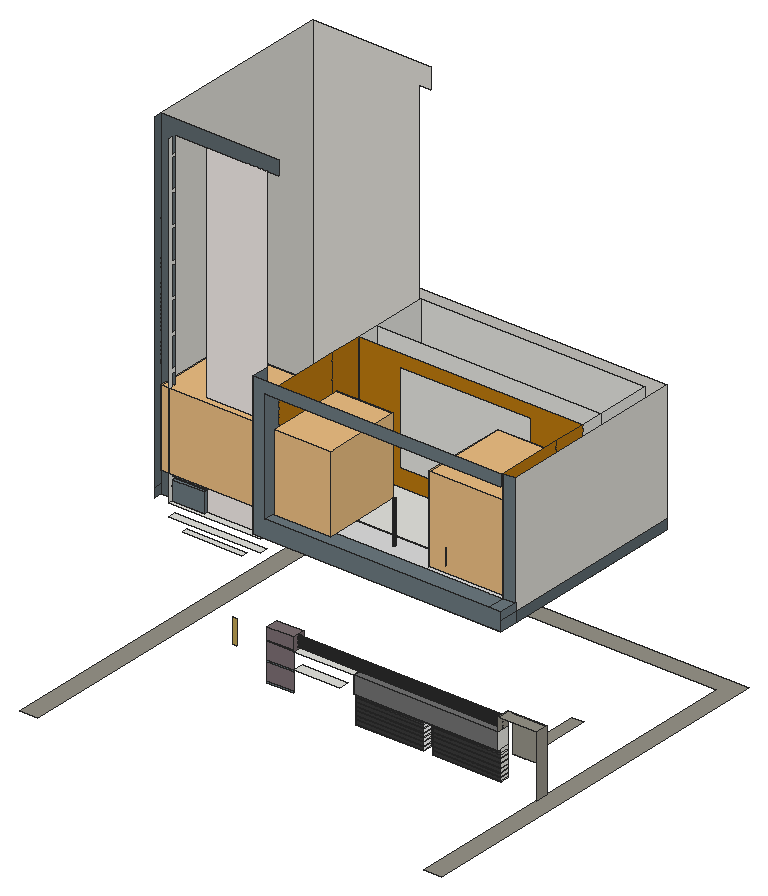
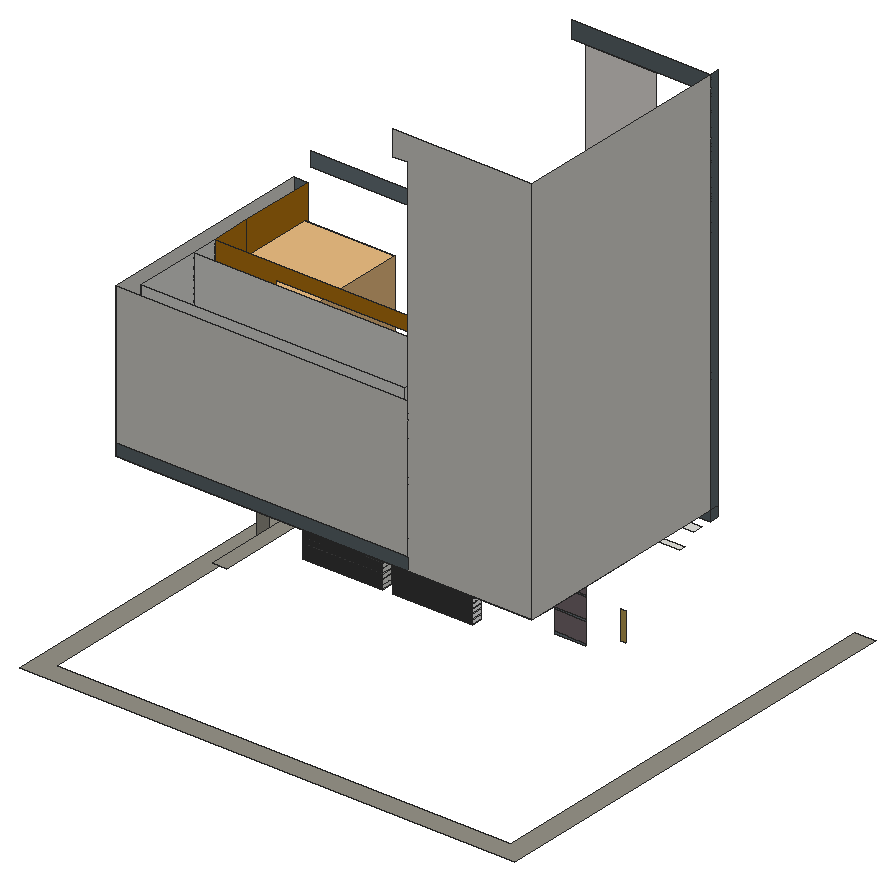
# SketchUp Ruby script. Lengths in inches.
U = 1.inch
M = Sketchup.active_model
def pt(a) = Geom::Point3d.new(a.map { |v| v * U })
def face(e, loops, mat)
  f = e.add_face(loops[0].map { |a| pt(a) })
  loops[1..].each { |l| e.add_face(l.map { |a| pt(a) }).erase! }
  f.material = f.back_material = mat if mat
  f
end
# faces: each face lists its corners as indices into pts; further lists are holes
def faces(e, pts, list, mat = nil) = list.each { |f| face(e, (f[0].is_a?(Array) ? f : [f]).map { |l| l.map { |i| pts[i] } }, mat) }
# xy, xz, yz: faces in a plane at the given z, y or x. An outline is a flat list of corners, or four numbers for a rectangle; further outlines are holes
def ring(l) = l.size == 4 ? [[l[0], l[1]], [l[2], l[1]], [l[2], l[3]], [l[0], l[3]]] : l.each_slice(2).to_a
def flat(e, list, mat, &to3) = list.each { |f| face(e, (f[0].is_a?(Array) ? f : [f]).map { |l| ring(l).map { |u, v| to3.(u, v) } }, mat) }
def xy(e, z, list, mat = nil) = flat(e, list, mat) { |x, y| [x, y, z] }
def xz(e, y, list, mat = nil) = flat(e, list, mat) { |x, z| [x, y, z] }
def yz(e, x, list, mat = nil) = flat(e, list, mat) { |y, z| [x, y, z] }
def lines(e, pts, list) = list.each { |a, b| e.add_line(pt(pts[a]), pt(pts[b])) }
# prism: a flat outline (further loops are holes) pulled along v
def prism(e, loops, v, mat = nil)
  f = face(e, loops, mat); d = Geom::Vector3d.new(v.map { |x| x * U })
  f.pushpull(f.normal.samedirection?(d) ? d.length : -d.length)
end
def box(e, o, s, mat = nil) = prism(e, [[o, [o[0] + s[0], o[1], o[2]], [o[0] + s[0], o[1] + s[1], o[2]], [o[0], o[1] + s[1], o[2]]]], [0, 0, s[2]], mat)
def at(x, y, z, deg = 0) = Geom::Transformation.translation(pt([x, y, z])) * Geom::Transformation.rotation(ORIGIN, Z_AXIS, deg.degrees)
def axes(o, x, y, z) = Geom::Transformation.new([*x, 0, *y, 0, *z, 0, *pt(o).to_a, 1])
def part(name) = M.definitions.add(name)
# library, detail: a bought-in or finely detailed component or shape, given as its bounding box
def library(name, o, s) = part(name).tap { |d| box(d.entities, o, s) }
def detail(e, o, s) = box(e.add_group.entities, o, s)
def put(e, d, t, mat = nil) = e.add_instance(d, t).tap { |i| i.material = mat if mat }
def group(e, t, mat = nil) = e.add_group.tap { |g| g.transformation = t; g.material = mat if mat }.entities
root = M.entities
M.materials.add("[0130_Gainsboro]").color = [220, 220, 220]
M.materials.add("[Asphalt New]").color = [124, 111, 115]
M.materials.add("[Blinds Cloth Horizontal]").color = [192, 163, 85]
M.materials.add("[Blinds Wood Light]").color = [186, 120, 16]
M.materials.add("[Color M00]").color = [255, 255, 255]
M.materials.add("[Color M05]").color = [114, 114, 114]
M.materials.add("[Color M06]").color = [86, 86, 86]
M.materials.add("[Color M07]").color = [58, 58, 58]
M.materials.add("[Formica Graystone]").color = [149, 146, 135]
M.materials.add("[Formica Laminate Dark]").color = [50, 53, 60]
M.materials.add("[Formica Speckled Grey]").color = [107, 120, 127]
M.materials.add("[Formica Speckled Grey]1").color = [94, 105, 111]
M.materials.add("[Terrazzo Tile Light]").color = [219, 217, 210]
M.materials.add("[White Square Tile]").color = [240, 234, 230]
c1 = library("chau cay",[-24.34,-109.24,0],[56.46,62.58,79.69])
c2 = library("Sem+nome",[-20.92,-6.25,0],[92.79,42.83,52.11])
xy(root,41.8125,[[0,0,9.63,0,9.63,200.71,221.32,200.71,221.32,0,230.95,0,230.95,210.34,0,210.34]],"[Formica Graystone]")
xy(root,42.59,[[200.125,79.26,200.1875,83.94]])
xy(root,42.59,[[162.78,79.26,200.125,83.94]],"[Color M07]")
xy(root,42.84,[[120.8,79.26,158.09,83.94]],"[Color M07]")
xy(root,42.9,[[162.78,79.26,200.125,83.94]],"[Color M07]")
xy(root,43.27,[[120.8,79.26,158.09,83.94]],"[Color M07]")
xy(root,44.66,[[162.78,79.26,200.125,83.94]],"[Color M07]")
xy(root,44.96,[[162.78,79.26,200.125,83.94]],"[Color M07]")
xy(root,45.03,[[120.8,79.26,158.09,83.94]],"[Color M07]")
xy(root,45.46,[[120.8,79.26,158.09,83.94]],"[Color M07]")
xy(root,46.72,[[162.78,79.26,200.125,83.94]],"[Color M07]")
xy(root,47.21,[[162.78,79.26,200.125,83.94]],"[Color M07]")
xy(root,47.22,[[120.8,79.26,158.09,83.94]],"[Color M07]")
xy(root,47.65,[[120.8,79.26,158.09,83.94]],"[Color M07]")
xy(root,48.97,[[162.78,79.26,200.125,83.94]],"[Color M07]")
xy(root,49.41,[[120.8,79.26,158.09,83.94]],"[Color M07]")
xy(root,49.59,[[162.78,79.26,200.125,83.94]],"[Color M07]")
xy(root,49.84,[[120.8,79.26,158.09,83.94]],"[Color M07]")
xy(root,51.34,[[162.78,79.26,200.125,83.94]],"[Color M07]")
xy(root,51.59,[[120.8,79.26,158.09,83.94]],"[Color M07]")
xy(root,51.96,[[162.78,79.26,200.125,83.94]],"[Color M07]")
xy(root,52.02,[[120.8,79.26,158.09,83.94]],"[Color M07]")
xy(root,53.72,[[162.78,79.26,200.125,83.94]],"[Color M07]")
xy(root,53.78,[[120.8,79.26,158.09,83.94]],"[Color M07]")
xy(root,54.21,[[120.8,79.26,158.09,83.94],[162.78,79.26,200.125,83.94]],"[Color M07]")
xy(root,55.3125,[[202.93,83.94,209.59,124.55]],"[Formica Graystone]")
xy(root,55.97,[[120.8,79.26,158.09,83.94],[162.78,79.26,200.125,83.94]],"[Color M07]")
xy(root,56.67,[[120.8,79.26,158.09,83.94],[162.78,79.26,200.125,83.94]],"[Color M07]")
xy(root,58.88,[[88.1,77.29,113.16,83.29],[120.8,79.26,158.09,83.94],[162.78,79.26,200.125,83.94]])
xy(root,58.88,[[120.8,77.29,200.125,79.26]],"[Color M05]")
xy(root,68,[[88.1,77.29,120.8,83.94]])
xy(root,68,[[120.8,77.29,200.125,83.94]],"[Color M05]")
xy(root,75.3125,[[73.48,77.29,88.1,83.94]],"[Asphalt New]")
xy(root,75.3125,[[200.125,77.29,221.32,83.94]],"[Formica Graystone]")
xy(root,105.34,[[27.2,77.29,59.83,80.42]])
xy(root,112.0625,[[97.58,124.55,186.72,127.86]])
xy(root,113.3,[[22.92,72.92,73.48,77.29]])
xy(root,120,[[22.92,72.92,73.48,72.92,73.48,77.29,40.57,77.29,40.57,75.48,22.92,75.48],[22.92,75.48,40.57,77.29]])
xy(root,124.8125,[[90.48,86.18,89.1875,86.35,87.98,86.85,86.95,87.65,86.15,88.68,85.65,89.89,85.48,91.18,85.65,92.48,86.15,93.68,86.95,94.72,87.98,95.51,89.1875,96.01,90.48,96.18,91.78,96.01,92.98,95.51,94.02,94.72,94.8125,93.68,95.3125,92.48,95.48,91.18,95.3125,89.89,94.8125,88.68,94.02,87.65,92.98,86.85,91.78,86.35],[138.67,86.18,137.375,86.35,136.17,86.85,135.13,87.65,134.34,88.68,133.84,89.89,133.67,91.18,133.84,92.48,134.34,93.68,135.13,94.72,136.17,95.51,137.375,96.01,138.67,96.18,139.96,96.01,141.17,95.51,142.21,94.72,143,93.68,143.5,92.48,143.67,91.18,143.5,89.89,143,88.68,142.21,87.65,141.17,86.85,139.96,86.35],[185.98,86.18,184.6875,86.35,183.48,86.85,182.45,87.65,181.65,88.68,181.15,89.89,180.98,91.18,181.15,92.48,181.65,93.68,182.45,94.72,183.48,95.51,184.6875,96.01,185.98,96.18,187.28,96.01,188.48,95.51,189.52,94.72,190.3125,93.68,190.8125,92.48,190.98,91.18,190.8125,89.89,190.3125,88.68,189.52,87.65,188.48,86.85,187.28,86.35],[15.28,124.55,21.94,129.24],[21.94,124.55,202.93,129.24],
  [202.93,124.55,209.59,129.24],[15.28,129.24,21.94,174.54],[21.94,129.24,202.93,174.54],[202.93,129.24,209.59,181.19],[15.28,174.54,202.93,181.19]])
xy(root,124.8125,[[73.48,67.6,209.59,77.29]],"[Formica Speckled Grey]")
xy(root,124.8125,[[[73.48,77.29,209.59,124.55],[90.48,86.18,91.78,86.35,92.98,86.85,94.02,87.65,94.8125,88.68,95.3125,89.89,95.48,91.18,95.3125,92.48,94.8125,93.68,94.02,94.72,92.98,95.51,91.78,96.01,90.48,96.18,89.1875,96.01,87.98,95.51,86.95,94.72,86.15,93.68,85.65,92.48,85.48,91.18,85.65,89.89,86.15,88.68,86.95,87.65,87.98,86.85,89.1875,86.35],[185.98,86.18,187.28,86.35,188.48,86.85,189.52,87.65,190.3125,88.68,190.8125,89.89,190.98,91.18,190.8125,92.48,190.3125,93.68,189.52,94.72,188.48,95.51,187.28,96.01,185.98,96.18,184.6875,96.01,183.48,95.51,182.45,94.72,181.65,93.68,181.15,92.48,180.98,91.18,181.15,89.89,181.65,88.68,182.45,87.65,183.48,86.85,184.6875,86.35],[138.67,86.18,139.96,86.35,141.17,86.85,142.21,87.65,143,88.68,143.5,89.89,143.67,91.18,143.5,92.48,143,93.68,142.21,94.72,141.17,95.51,139.96,96.01,138.67,96.18,137.375,96.01,136.17,95.51,135.13,94.72,134.34,93.68,133.84,92.48,133.67,91.18,133.84,89.89,134.34,88.68,135.13,87.65,136.17,86.85,137.375,86.35]]],"[Formica Speckled Grey]1")
xy(root,130.3125,[[80.125,91.25,202.95,131.65],[80.125,131.65,202.95,143.96],[80.125,143.96,202.95,174.55]])
xy(root,130.5,[[22.92,75.48,40.57,77.29]],"[Formica Speckled Grey]")
xy(root,132.27,[[22.92,75.48,40.57,77.29]],"[Formica Speckled Grey]")
xy(root,134.5,[[104.45,84,104.25,84.02,104.07,84.1,103.92,84.22,103.8,84.375,103.72,84.55,103.7,84.75,103.72,84.94,103.8,85.125,103.92,85.28,104.07,85.4,104.25,85.47,104.45,85.5,104.64,85.47,104.82,85.4,104.98,85.28,105.1,85.125,105.17,84.94,105.2,84.75,105.17,84.55,105.1,84.375,104.98,84.22,104.82,84.1,104.64,84.02],[137.32,84,137.13,84.02,136.95,84.1,136.79,84.22,136.67,84.375,136.6,84.55,136.57,84.75,136.6,84.94,136.67,85.125,136.79,85.28,136.95,85.4,137.13,85.47,137.32,85.5,137.52,85.47,137.7,85.4,137.85,85.28,137.97,85.125,138.05,84.94,138.07,84.75,138.05,84.55,137.97,84.375,137.85,84.22,137.7,84.1,137.52,84.02],[166.51,84,166.32,84.02,166.13,84.1,165.98,84.22,165.86,84.375,165.79,84.55,165.76,84.75,165.79,84.94,165.86,85.125,165.98,85.28,166.13,85.4,166.32,85.47,166.51,85.5,166.7,85.47,166.88,85.4,167.04,85.28,167.16,85.125,167.23,84.94,167.26,84.75,167.23,84.55,167.16,84.375,167.04,84.22,166.88,84.1,166.7,84.02]])
xy(root,134.5,[[[80.125,77.29,202.95,91.25],[166.51,84,166.32,84.02,166.13,84.1,165.98,84.22,165.86,84.375,165.79,84.55,165.76,84.75,165.79,84.94,165.86,85.125,165.98,85.28,166.13,85.4,166.32,85.47,166.51,85.5,166.7,85.47,166.88,85.4,167.04,85.28,167.16,85.125,167.23,84.94,167.26,84.75,167.23,84.55,167.16,84.375,167.04,84.22,166.88,84.1,166.7,84.02],[137.32,84,137.13,84.02,136.95,84.1,136.79,84.22,136.67,84.375,136.6,84.55,136.57,84.75,136.6,84.94,136.67,85.125,136.79,85.28,136.95,85.4,137.13,85.47,137.32,85.5,137.52,85.47,137.7,85.4,137.85,85.28,137.97,85.125,138.05,84.94,138.07,84.75,138.05,84.55,137.97,84.375,137.85,84.22,137.7,84.1,137.52,84.02],[104.45,84,104.25,84.02,104.07,84.1,103.92,84.22,103.8,84.375,103.72,84.55,103.7,84.75,103.72,84.94,103.8,85.125,103.92,85.28,104.07,85.4,104.25,85.47,104.45,85.5,104.64,85.47,104.82,85.4,104.98,85.28,105.1,85.125,105.17,84.94,105.2,84.75,105.17,84.55,105.1,84.375,104.98,84.22,104.82,84.1,104.64,84.02]]],"[0130_Gainsboro]")
xy(root,134.5,[[80.125,67.6,202.95,77.29],[202.95,67.6,209.59,77.29]],"[Formica Speckled Grey]")
xz(root,67.6,[[73.48,124.8125,209.59,124.8125,209.59,134.5,80.125,134.5,80.125,195.875,209.59,195.875,209.59,202.375,73.48,202.375]],"[Formica Speckled Grey]")
xz(root,75.48,[[22.92,120,40.57,130.5],[22.92,132.27,40.57,146.25]],"[Formica Speckled Grey]")
xz(root,77.29,[[22.92,120,40.57,130.5],[22.92,132.27,40.57,146.25]])
xz(root,77.29,[[73.48,48.75,88.1,57.875],[73.48,58.88,88.1,68],[73.48,68.86,88.1,75.3125]],"[Asphalt New]")
xz(root,77.29,[[120.8,58.88,200.125,68]],"[Color M05]")
xz(root,77.29,[[22.92,130.5,40.57,132.27]],"[Formica Laminate Dark]")
xz(root,77.29,[[73.48,47.5625,88.1,48.75],[73.48,57.875,88.1,58.88],[73.48,68,88.1,68.86],[202.95,134.5,209.59,195.875]],"[Formica Speckled Grey]")
xz(root,77.29,[[15.28,120,15.28,306.8125,80.125,306.8125,80.125,298.85,22.92,298.85,22.92,120]],"[Formica Speckled Grey]1")
xz(root,77.29,[[40.57,120,73.48,298.85]],"[White Square Tile]")
xz(root,79.26,[[162.78,42.9,200.125,44.66],[120.8,43.27,158.09,45.03],[162.78,44.96,200.125,46.72],[120.8,45.46,158.09,47.22],[162.78,47.21,200.125,48.97],
  [120.8,47.65,158.09,49.41],[162.78,49.59,200.125,51.34],[120.8,49.84,158.09,51.59],[162.78,51.96,200.125,53.72],[120.8,52.02,158.09,53.78],
  [120.8,54.21,158.09,55.97],[162.78,54.21,200.125,55.97],[120.8,56.67,158.09,58.88],[162.78,56.67,200.125,58.88]],"[Color M07]")
xz(root,80.42,[[52.45,57.88,54.7,71.19]],"[Blinds Cloth Horizontal]")
xz(root,83.94,[[120.8,58.88,200.125,68]],"[Color M05]")
xz(root,83.94,[[162.78,42.9,200.125,44.66],[120.8,43.27,158.09,45.03],[162.78,44.96,200.125,46.72],[120.8,45.46,158.09,47.22],[162.78,47.21,200.125,48.97],
  [120.8,47.65,158.09,49.41],[162.78,49.59,200.125,51.34],[120.8,49.84,158.09,51.59],[162.78,51.96,200.125,53.72],[120.8,52.02,158.09,53.78],
  [120.8,54.21,158.09,55.97],[162.78,54.21,200.125,55.97],[120.8,56.67,158.09,58.88],[162.78,56.67,200.125,58.88]],"[Color M07]")
xz(root,83.94,[[202.93,55.3125,221.32,75.3125]],"[Formica Graystone]")
xz(root,91.25,[[80.125,130.3125,202.95,134.5]])
xz(root,131.65,[[[80.125,130.3125,202.95,195.875],[102.7,139.62,174.38,189.18]]],"[Blinds Wood Light]")
xz(root,143.96,[[80.125,130.3125,202.95,195.875]])
xz(root,174.55,[[80.125,130.3125,202.95,195.875]])
xz(root,181.19,[[73.48,124.8125,209.59,130.3125]],"[Formica Speckled Grey]1")
xz(root,181.19,[[15.28,124.8125,15.28,306.8125,80.125,306.8125,80.125,295.4375,73.48,295.4375,73.48,124.8125],[73.48,130.3125,209.59,195.875]],"[Terrazzo Tile Light]")
yz(root,15.28,[[72.92,120,77.29,124.8125],[72.92,124.8125,77.29,306.8125]],"[Formica Speckled Grey]1")
yz(root,15.28,[[77.29,124.8125,181.19,306.8125]],"[Terrazzo Tile Light]")
yz(root,22.92,[[72.92,120,75.48,120,75.48,130.5,77.29,130.5,77.29,132.27,75.48,132.27,75.48,146.25,77.29,146.25,77.29,148.25,75.48,148.25,75.48,164,77.29,164,77.29,166.81,75.48,166.81,75.48,182.5625,77.29,182.5625,77.29,184.81,75.48,184.81,75.48,200.5625,77.29,200.5625,77.29,202.43,75.48,202.43,75.48,218.1875,77.29,218.1875,77.29,220,75.48,220,75.48,235.75,77.29,235.75,77.29,237.75,75.48,237.75,75.48,253.5,77.29,253.5,77.29,255.31,75.48,255.31,75.48,271.0625,77.29,271.0625,77.29,272.68,75.48,272.68,75.48,288.4375,77.29,288.4375,77.29,290.11,75.48,290.11,75.48,298.85,72.92,298.85],[75.48,132.27,77.29,146.25]])
yz(root,22.92,[[75.48,120,77.29,130.5]],"[Formica Speckled Grey]1")
yz(root,40.57,[[75.48,120,77.29,130.5],[75.48,132.27,77.29,146.25]],"[Formica Speckled Grey]")
yz(root,73.48,[[67.6,124.8125,77.29,202.375]],"[Formica Speckled Grey]")
yz(root,80.125,[[131.65,130.3125,143.96,195.875],[143.96,130.3125,174.55,195.875]])
yz(root,80.125,[[91.25,130.3125,131.65,130.3125,131.65,195.875,113.38,195.875,113.38,134.5,91.25,134.5],[[77.29,134.5,113.38,195.875],[84.34,157.04,84.16,157.06,83.99,157.13,83.85,157.24,83.74,157.38,83.67,157.54,83.65,157.72,83.67,157.9,83.74,158.07,83.85,158.21,83.99,158.32,84.16,158.39,84.34,158.41,84.51,158.39,84.68,158.32,84.82,158.21,84.93,158.07,85,157.9,85.02,157.72,85,157.54,84.93,157.38,84.82,157.24,84.68,157.13,84.51,157.06],[84.34,151.97,84.16,152,83.99,152.06,83.85,152.17,83.74,152.32,83.67,152.48,83.65,152.66,83.67,152.84,83.74,153,83.85,153.15,83.99,153.26,84.16,153.32,84.34,153.35,84.51,153.32,84.68,153.26,84.82,153.15,84.93,153,85,152.84,85.02,152.66,85,152.48,84.93,152.32,84.82,152.17,84.68,152.06,84.51,152],[84.34,154.47,84.16,154.5,83.99,154.56,83.85,154.67,83.74,154.82,83.67,154.98,83.65,155.16,83.67,155.34,83.74,155.5,83.85,155.65,83.99,155.76,84.16,155.82,84.34,155.85,84.51,155.82,84.68,155.76,84.82,155.65,84.93,155.5,85,155.34,85.02,155.16,85,154.98,84.93,154.82,84.82,154.67,84.68,154.56,84.51,154.5],[84.14,139.71,83.98,139.73,83.83,139.79,83.7,139.89,83.6,140.02,83.54,140.17,83.52,140.33,83.54,140.49,83.6,140.64,83.7,140.77,83.83,140.87,83.98,140.93,84.14,140.96,84.3,140.93,84.45,140.87,84.58,140.77,84.68,140.64,84.74,140.49,84.77,140.33,84.74,140.17,84.68,140.02,84.58,139.89,84.45,139.79,84.3,139.73],[84.14,142.77,83.98,142.79,83.83,142.85,83.7,142.95,83.6,143.08,83.54,143.23,83.52,143.39,83.54,143.56,83.6,143.71,83.7,143.84,83.83,143.93,83.98,144,84.14,144.02,84.3,144,84.45,143.93,84.58,143.84,84.68,143.71,84.74,143.56,84.77,143.39,84.74,143.23,84.68,143.08,84.58,142.95,84.45,142.85,84.3,142.79],[84.31,136.76,84.15,136.78,84,136.84,83.87,136.94,83.77,137.07,83.7,137.22,83.68,137.39,83.7,137.55,83.77,137.7,83.87,137.83,84,137.93,84.15,137.99,84.31,138.01,84.47,137.99,84.62,137.93,84.75,137.83,84.85,137.7,84.91,137.55,84.93,137.39,84.91,137.22,84.85,137.07,84.75,136.94,84.62,136.84,84.47,136.78],[84.31,145.95,84.15,145.97,84,146.03,83.87,146.13,83.77,146.26,83.7,146.41,83.68,146.57,83.7,146.74,83.77,146.89,83.87,147.02,84,147.11,84.15,147.18,84.31,147.2,84.47,147.18,84.62,147.11,84.75,147.02,84.85,146.89,84.91,146.74,84.93,146.57,84.91,146.41,84.85,146.26,84.75,146.13,84.62,146.03,84.47,145.97],[84.31,149.39,84.15,149.41,84,149.47,83.87,149.57,83.77,149.7,83.7,149.85,83.68,150.01,83.7,150.17,83.77,150.32,83.87,150.45,84,150.55,84.15,150.61,84.31,150.64,84.47,150.61,84.62,150.55,84.75,150.45,84.85,150.32,84.91,150.17,84.93,150.01,84.91,149.85,84.85,149.7,84.75,149.57,84.62,149.47,84.47,149.41]]],"[Blinds Wood Light]")
yz(root,80.125,[[67.6,134.5,77.29,195.875]],"[Formica Speckled Grey]")
yz(root,88.1,[[80.61,68.75,80.4375,68.78,80.27,68.84,80.13,68.95,80.02,69.1,79.95,69.26,79.93,69.4375,79.95,69.62,80.02,69.78,80.13,69.93,80.27,70.03,80.4375,70.1,80.61,70.125,80.79,70.1,80.96,70.03,81.1,69.93,81.21,69.78,81.28,69.62,81.3,69.4375,81.28,69.26,81.21,69.1,81.1,68.95,80.96,68.84,80.79,68.78],[80.51,70.85,80.33,70.875,80.17,70.94,80.02,71.05,79.91,71.19,79.85,71.36,79.82,71.54,79.85,71.72,79.91,71.88,80.02,72.02,80.17,72.13,80.33,72.2,80.51,72.23,80.6875,72.2,80.85,72.13,81,72.02,81.1,71.88,81.17,71.72,81.2,71.54,81.17,71.36,81.1,71.19,81,71.05,80.85,70.94,80.6875,70.875],[80.48,72.98,80.25,73.01,80.04,73.1,79.86,73.24,79.72,73.42,79.64,73.63,79.61,73.86,79.64,74.08,79.72,74.3,79.86,74.48,80.04,74.62,80.25,74.7,80.48,74.73,80.71,74.7,80.92,74.62,81.1,74.48,81.24,74.3,81.33,74.08,81.36,73.86,81.33,73.63,81.24,73.42,81.1,73.24,80.92,73.1,80.71,73.01]])
yz(root,88.1,[[[77.29,68,83.94,75.3125],[80.48,72.98,80.25,73.01,80.04,73.1,79.86,73.24,79.72,73.42,79.64,73.63,79.61,73.86,79.64,74.08,79.72,74.3,79.86,74.48,80.04,74.62,80.25,74.7,80.48,74.73,80.71,74.7,80.92,74.62,81.1,74.48,81.24,74.3,81.33,74.08,81.36,73.86,81.33,73.63,81.24,73.42,81.1,73.24,80.92,73.1,80.71,73.01],[80.61,68.75,80.4375,68.78,80.27,68.84,80.13,68.95,80.02,69.1,79.95,69.26,79.93,69.4375,79.95,69.62,80.02,69.78,80.13,69.93,80.27,70.03,80.4375,70.1,80.61,70.125,80.79,70.1,80.96,70.03,81.1,69.93,81.21,69.78,81.28,69.62,81.3,69.4375,81.28,69.26,81.21,69.1,81.1,68.95,80.96,68.84,80.79,68.78],[80.51,70.85,80.33,70.875,80.17,70.94,80.02,71.05,79.91,71.19,79.85,71.36,79.82,71.54,79.85,71.72,79.91,71.88,80.02,72.02,80.17,72.13,80.33,72.2,80.51,72.23,80.6875,72.2,80.85,72.13,81,72.02,81.1,71.88,81.17,71.72,81.2,71.54,81.17,71.36,81.1,71.19,81,71.05,80.85,70.94,80.6875,70.875]]],"[Asphalt New]")
yz(root,120.8,[[79.26,42.84,83.94,43.27],[79.26,45.03,83.94,45.46],[79.26,47.22,83.94,47.65],[79.26,49.41,83.94,49.84],[79.26,51.59,83.94,52.02],
  [79.26,53.78,83.94,54.21],[79.26,55.97,83.94,56.67],[77.29,58.88,83.94,68]])
yz(root,120.8,[[79.26,43.27,83.94,45.03],[79.26,45.46,83.94,47.22],[79.26,47.65,83.94,49.41],[79.26,49.84,83.94,51.59],[79.26,52.02,83.94,53.78],
  [79.26,54.21,83.94,55.97]],"[Color M00]")
yz(root,158.09,[[79.26,42.84,83.94,43.27],[79.26,45.03,83.94,45.46],[79.26,47.22,83.94,47.65],[79.26,49.41,83.94,49.84],[79.26,51.59,83.94,52.02],
  [79.26,53.78,83.94,54.21],[79.26,55.97,83.94,56.67],[79.26,56.67,83.94,58.88]])
yz(root,158.09,[[79.26,43.27,83.94,45.03],[79.26,45.46,83.94,47.22],[79.26,47.65,83.94,49.41],[79.26,49.84,83.94,51.59],[79.26,52.02,83.94,53.78],
  [79.26,54.21,83.94,55.97]],"[Color M00]")
yz(root,162.78,[[79.26,42.59,83.94,42.9],[79.26,42.9,83.94,44.66],[79.26,44.66,83.94,44.96],[79.26,44.96,83.94,46.72],[79.26,46.72,83.94,47.21],
  [79.26,47.21,83.94,48.97],[79.26,48.97,83.94,49.59],[79.26,49.59,83.94,51.34],[79.26,51.34,83.94,51.96],[79.26,51.96,83.94,53.72],
  [79.26,53.72,83.94,54.21],[79.26,54.21,83.94,55.97],[79.26,55.97,83.94,56.67]])
yz(root,200.125,[[79.26,42.59,83.94,42.9],[79.26,42.9,83.94,44.66],[79.26,44.66,83.94,44.96],[79.26,44.96,83.94,46.72],[79.26,46.72,83.94,47.21],
  [79.26,47.21,83.94,48.97],[79.26,48.97,83.94,49.59],[79.26,49.59,83.94,51.34],[79.26,51.34,83.94,51.96],[79.26,51.96,83.94,53.72],
  [79.26,53.72,83.94,54.21],[79.26,54.21,83.94,55.97],[79.26,55.97,83.94,56.67],[79.26,56.67,83.94,58.88],[77.29,58.88,83.94,68]])
yz(root,200.125,[[[77.29,68,83.94,75.3125],[80.48,72.98,80.71,73.01,80.92,73.1,81.1,73.24,81.24,73.42,81.33,73.63,81.36,73.86,81.33,74.08,81.24,74.3,81.1,74.48,80.92,74.62,80.71,74.7,80.48,74.73,80.25,74.7,80.04,74.62,79.86,74.48,79.72,74.3,79.64,74.08,79.61,73.86,79.64,73.63,79.72,73.42,79.86,73.24,80.04,73.1,80.25,73.01],[80.61,68.75,80.79,68.78,80.96,68.84,81.1,68.95,81.21,69.1,81.28,69.26,81.3,69.4375,81.28,69.62,81.21,69.78,81.1,69.93,80.96,70.03,80.79,70.1,80.61,70.125,80.4375,70.1,80.27,70.03,80.13,69.93,80.02,69.78,79.95,69.62,79.93,69.4375,79.95,69.26,80.02,69.1,80.13,68.95,80.27,68.84,80.4375,68.78],[80.51,70.85,80.6875,70.875,80.85,70.94,81,71.05,81.1,71.19,81.17,71.36,81.2,71.54,81.17,71.72,81.1,71.88,81,72.02,80.85,72.13,80.6875,72.2,80.51,72.23,80.33,72.2,80.17,72.13,80.02,72.02,79.91,71.88,79.85,71.72,79.82,71.54,79.85,71.36,79.91,71.19,80.02,71.05,80.17,70.94,80.33,70.875]]],"[Formica Graystone]")
yz(root,202.95,[[131.65,130.3125,143.96,195.875],[143.96,130.3125,174.55,195.875]])
yz(root,202.95,[[91.25,130.3125,91.25,134.5,113.38,134.5,113.38,195.875,131.65,195.875,131.65,130.3125],[[77.29,134.5,113.38,195.875],[84.34,154.47,84.51,154.5,84.68,154.56,84.82,154.67,84.93,154.82,85,154.98,85.02,155.16,85,155.34,84.93,155.5,84.82,155.65,84.68,155.76,84.51,155.82,84.34,155.85,84.16,155.82,83.99,155.76,83.85,155.65,83.74,155.5,83.67,155.34,83.65,155.16,83.67,154.98,83.74,154.82,83.85,154.67,83.99,154.56,84.16,154.5],[84.34,157.04,84.51,157.06,84.68,157.13,84.82,157.24,84.93,157.38,85,157.54,85.02,157.72,85,157.9,84.93,158.07,84.82,158.21,84.68,158.32,84.51,158.39,84.34,158.41,84.16,158.39,83.99,158.32,83.85,158.21,83.74,158.07,83.67,157.9,83.65,157.72,83.67,157.54,83.74,157.38,83.85,157.24,83.99,157.13,84.16,157.06],[84.34,151.97,84.51,152,84.68,152.06,84.82,152.17,84.93,152.32,85,152.48,85.02,152.66,85,152.84,84.93,153,84.82,153.15,84.68,153.26,84.51,153.32,84.34,153.35,84.16,153.32,83.99,153.26,83.85,153.15,83.74,153,83.67,152.84,83.65,152.66,83.67,152.48,83.74,152.32,83.85,152.17,83.99,152.06,84.16,152],[84.14,142.77,84.3,142.79,84.45,142.85,84.58,142.95,84.68,143.08,84.74,143.23,84.77,143.39,84.74,143.56,84.68,143.71,84.58,143.84,84.45,143.93,84.3,144,84.14,144.02,83.98,144,83.83,143.93,83.7,143.84,83.6,143.71,83.54,143.56,83.52,143.39,83.54,143.23,83.6,143.08,83.7,142.95,83.83,142.85,83.98,142.79],[84.14,139.71,84.3,139.73,84.45,139.79,84.58,139.89,84.68,140.02,84.74,140.17,84.77,140.33,84.74,140.49,84.68,140.64,84.58,140.77,84.45,140.87,84.3,140.93,84.14,140.96,83.98,140.93,83.83,140.87,83.7,140.77,83.6,140.64,83.54,140.49,83.52,140.33,83.54,140.17,83.6,140.02,83.7,139.89,83.83,139.79,83.98,139.73],[84.31,145.95,84.47,145.97,84.62,146.03,84.75,146.13,84.85,146.26,84.91,146.41,84.93,146.57,84.91,146.74,84.85,146.89,84.75,147.02,84.62,147.11,84.47,147.18,84.31,147.2,84.15,147.18,84,147.11,83.87,147.02,83.77,146.89,83.7,146.74,83.68,146.57,83.7,146.41,83.77,146.26,83.87,146.13,84,146.03,84.15,145.97],[84.31,149.39,84.47,149.41,84.62,149.47,84.75,149.57,84.85,149.7,84.91,149.85,84.93,150.01,84.91,150.17,84.85,150.32,84.75,150.45,84.62,150.55,84.47,150.61,84.31,150.64,84.15,150.61,84,150.55,83.87,150.45,83.77,150.32,83.7,150.17,83.68,150.01,83.7,149.85,83.77,149.7,83.87,149.57,84,149.47,84.15,149.41],[84.31,136.76,84.47,136.78,84.62,136.84,84.75,136.94,84.85,137.07,84.91,137.22,84.93,137.39,84.91,137.55,84.85,137.7,84.75,137.83,84.62,137.93,84.47,137.99,84.31,138.01,84.15,137.99,84,137.93,83.87,137.83,83.77,137.7,83.7,137.55,83.68,137.39,83.7,137.22,83.77,137.07,83.87,136.94,84,136.84,84.15,136.78]]],"[Blinds Wood Light]")
yz(root,209.59,[[67.6,124.8125,77.29,130.3125],[67.6,130.3125,77.29,134.5]],"[Formica Speckled Grey]")
yz(root,209.59,[[77.29,124.8125,181.19,130.3125]],"[Formica Speckled Grey]1")
yz(root,209.59,[[77.29,130.3125,181.19,195.875]],"[Terrazzo Tile Light]")
yz(root,221.32,[[77.29,41.8125,83.94,75.3125]],"[Formica Graystone]")
p = [[88.1,80.13,68.95],[88.1,80.27,68.84],[200.125,80.27,68.84],[200.125,80.13,68.95],[88.1,80.4375,68.78],[200.125,80.4375,68.78],
  [88.1,80.61,68.75],[200.125,80.61,68.75],[88.1,80.79,68.78],[200.125,80.79,68.78],[88.1,80.96,68.84],[200.125,80.96,68.84],
  [88.1,81.1,68.95],[200.125,81.1,68.95],[88.1,80.02,69.1],[200.125,80.02,69.1],[88.1,81.21,69.1],[200.125,81.21,69.1],
  [88.1,79.95,69.26],[200.125,79.95,69.26],[88.1,81.28,69.26],[200.125,81.28,69.26],[88.1,79.93,69.4375],[200.125,79.93,69.4375],
  [88.1,81.3,69.4375],[200.125,81.3,69.4375],[88.1,79.95,69.62],[200.125,79.95,69.62],[88.1,81.28,69.62],[200.125,81.28,69.62],
  [88.1,80.02,69.78],[200.125,80.02,69.78],[88.1,81.21,69.78],[200.125,81.21,69.78],[88.1,80.13,69.93],[200.125,80.13,69.93],
  [88.1,81.1,69.93],[200.125,81.1,69.93],[88.1,80.27,70.03],[200.125,80.27,70.03],[88.1,80.96,70.03],[200.125,80.96,70.03],
  [88.1,80.4375,70.1],[200.125,80.4375,70.1],[88.1,80.79,70.1],[200.125,80.79,70.1],[88.1,80.61,70.125],[200.125,80.61,70.125],
  [88.1,80.02,71.05],[88.1,80.17,70.94],[200.125,80.17,70.94],[200.125,80.02,71.05],[88.1,80.33,70.875],[200.125,80.33,70.875],
  [88.1,80.51,70.85],[200.125,80.51,70.85],[88.1,80.6875,70.875],[200.125,80.6875,70.875],[88.1,80.85,70.94],[200.125,80.85,70.94],
  [88.1,81,71.05],[200.125,81,71.05],[88.1,79.91,71.19],[200.125,79.91,71.19],[88.1,81.1,71.19],[200.125,81.1,71.19],
  [88.1,79.85,71.36],[200.125,79.85,71.36],[88.1,81.17,71.36],[200.125,81.17,71.36],[88.1,79.82,71.54],[200.125,79.82,71.54],
  [88.1,81.2,71.54],[200.125,81.2,71.54],[88.1,79.85,71.72],[200.125,79.85,71.72],[88.1,81.17,71.72],[200.125,81.17,71.72],
  [88.1,79.91,71.88],[200.125,79.91,71.88],[88.1,81.1,71.88],[200.125,81.1,71.88],[88.1,80.02,72.02],[200.125,80.02,72.02],
  [88.1,81,72.02],[200.125,81,72.02],[88.1,80.17,72.13],[200.125,80.17,72.13],[88.1,80.85,72.13],[200.125,80.85,72.13],
  [88.1,80.33,72.2],[200.125,80.33,72.2],[88.1,80.6875,72.2],[200.125,80.6875,72.2],[88.1,80.51,72.23],[200.125,80.51,72.23],
  [88.1,80.04,73.1],[88.1,80.25,73.01],[200.125,80.25,73.01],[200.125,80.04,73.1],[88.1,80.48,72.98],[200.125,80.48,72.98],
  [88.1,80.71,73.01],[200.125,80.71,73.01],[88.1,80.92,73.1],[200.125,80.92,73.1],[88.1,79.86,73.24],[200.125,79.86,73.24],
  [88.1,81.1,73.24],[200.125,81.1,73.24],[88.1,79.72,73.42],[200.125,79.72,73.42],[88.1,81.24,73.42],[200.125,81.24,73.42],
  [88.1,79.64,73.63],[200.125,79.64,73.63],[88.1,81.33,73.63],[200.125,81.33,73.63],[88.1,79.61,73.86],[200.125,79.61,73.86],
  [88.1,81.36,73.86],[200.125,81.36,73.86],[88.1,79.64,74.08],[200.125,79.64,74.08],[88.1,81.33,74.08],[200.125,81.33,74.08],
  [88.1,79.72,74.3],[200.125,79.72,74.3],[88.1,81.24,74.3],[200.125,81.24,74.3],[88.1,79.86,74.48],[200.125,79.86,74.48],
  [88.1,81.1,74.48],[200.125,81.1,74.48],[88.1,80.04,74.62],[200.125,80.04,74.62],[88.1,80.92,74.62],[200.125,80.92,74.62],
  [88.1,80.25,74.7],[200.125,80.25,74.7],[88.1,80.71,74.7],[200.125,80.71,74.7],[88.1,80.48,74.73],[200.125,80.48,74.73],
  [104.07,84.1,134.5],[104.25,84.02,134.5],[104.25,84.02,157.3125],[104.07,84.1,157.3125],[104.45,84,134.5],[104.45,84,157.3125],
  [104.64,84.02,134.5],[104.64,84.02,157.3125],[104.82,84.1,134.5],[104.82,84.1,157.3125],[136.95,84.1,134.5],[137.13,84.02,134.5],
  [137.13,84.02,157.38],[136.95,84.1,157.38],[137.32,84,134.5],[137.32,84,157.38],[137.52,84.02,134.5],[137.52,84.02,157.38],
  [137.7,84.1,134.5],[137.7,84.1,157.38],[166.13,84.1,134.5],[166.32,84.02,134.5],[166.32,84.02,157.1875],[166.13,84.1,157.1875],
  [166.51,84,134.5],[166.51,84,157.1875],[166.7,84.02,134.5],[166.7,84.02,157.1875],[166.88,84.1,134.5],[166.88,84.1,157.1875],
  [103.92,84.22,134.5],[103.92,84.22,157.3125],[104.98,84.22,134.5],[104.98,84.22,157.3125],[136.79,84.22,134.5],[136.79,84.22,157.38],
  [137.85,84.22,134.5],[137.85,84.22,157.38],[165.98,84.22,134.5],[165.98,84.22,157.1875],[167.04,84.22,134.5],[167.04,84.22,157.1875],
  [103.8,84.375,134.5],[103.8,84.375,157.3125],[105.1,84.375,134.5],[105.1,84.375,157.3125],[136.67,84.375,134.5],[136.67,84.375,157.38],
  [137.97,84.375,134.5],[137.97,84.375,157.38],[165.86,84.375,134.5],[165.86,84.375,157.1875],[167.16,84.375,134.5],[167.16,84.375,157.1875],
  [103.72,84.55,134.5],[103.72,84.55,157.3125],[105.17,84.55,134.5],[105.17,84.55,157.3125],[136.6,84.55,134.5],[136.6,84.55,157.38],
  [138.05,84.55,134.5],[138.05,84.55,157.38],[165.79,84.55,134.5],[165.79,84.55,157.1875],[167.23,84.55,134.5],[167.23,84.55,157.1875],
  [103.7,84.75,134.5],[103.7,84.75,157.3125],[105.2,84.75,134.5],[105.2,84.75,157.3125],[136.57,84.75,134.5],[136.57,84.75,157.38],
  [138.07,84.75,134.5],[138.07,84.75,157.38],[165.76,84.75,134.5],[165.76,84.75,157.1875],[167.26,84.75,134.5],[167.26,84.75,157.1875],
  [103.72,84.94,134.5],[103.72,84.94,157.3125],[105.17,84.94,134.5],[105.17,84.94,157.3125],[136.6,84.94,134.5],[136.6,84.93,157.38],
  [136.6,84.94,157.38],[138.05,84.94,134.5],[138.05,84.94,157.38],[138.05,84.93,157.38],[165.79,84.94,134.5],[165.79,84.94,157.1875],
  [167.23,84.94,134.5],[167.23,84.94,157.1875],[103.8,85.125,134.5],[103.8,85.125,157.3125],[105.1,85.125,134.5],[105.1,85.125,157.3125],
  [136.67,85.125,134.5],[136.67,85.125,157.38],[137.97,85.125,134.5],[137.97,85.125,157.38],[165.86,85.125,134.5],[165.86,85.125,157.1875],
  [167.16,85.125,134.5],[167.16,85.125,157.1875],[103.92,85.28,134.5],[103.92,85.28,157.3125],[104.98,85.28,134.5],[104.98,85.28,157.3125],
  [136.79,85.28,134.5],[136.79,85.28,157.38],[137.85,85.28,134.5],[137.85,85.28,157.38],[165.98,85.28,134.5],[165.98,85.28,157.1875],
  [167.04,85.28,134.5],[167.04,85.28,157.1875],[104.07,85.4,134.5],[104.07,85.4,157.3125],[104.82,85.4,134.5],[104.82,85.4,157.3125],
  [136.95,85.4,134.5],[136.95,85.4,157.38],[137.7,85.4,134.5],[137.7,85.4,157.38],[166.13,85.4,134.5],[166.13,85.4,157.1875],
  [166.88,85.4,134.5],[166.88,85.4,157.1875],[104.25,85.47,134.5],[104.25,85.47,157.3125],[104.64,85.47,134.5],[104.64,85.47,157.3125],
  [137.13,85.47,134.5],[137.13,85.47,157.38],[137.52,85.47,134.5],[137.52,85.47,157.38],[166.32,85.47,134.5],[166.32,85.47,157.1875],
  [166.7,85.47,134.5],[166.7,85.47,157.1875],[104.45,85.5,134.5],[104.45,85.5,157.3125],[137.32,85.5,134.5],[137.32,85.5,157.38],
  [166.51,85.5,134.5],[166.51,85.5,157.1875],[21.94,124.55,124.8125],[21.94,83.94,124.8125],[21.94,77.29,124.8125],[20.35,77.29,120],
  [20.35,72.92,120]]
faces(root,p,[[0,1,2,3],[1,4,5,2],[4,6,7,5],[6,8,9,7],[8,10,11,9],[10,12,13,11],[14,0,3,15],[12,16,17,13],
  [18,14,15,19],[16,20,21,17],[22,18,19,23],[20,24,25,21],[26,22,23,27],[24,28,29,25],[30,26,27,31],[28,32,33,29],
  [34,30,31,35],[32,36,37,33],[38,34,35,39],[36,40,41,37],[42,38,39,43],[40,44,45,41],[46,42,43,47],[44,46,47,45],
  [48,49,50,51],[49,52,53,50],[52,54,55,53],[54,56,57,55],[56,58,59,57],[58,60,61,59],[62,48,51,63],[60,64,65,61],
  [66,62,63,67],[64,68,69,65],[70,66,67,71],[68,72,73,69],[74,70,71,75],[72,76,77,73],[78,74,75,79],[76,80,81,77],
  [82,78,79,83],[80,84,85,81],[86,82,83,87],[84,88,89,85],[90,86,87,91],[88,92,93,89],[94,90,91,95],[92,94,95,93],
  [96,97,98,99],[97,100,101,98],[100,102,103,101],[102,104,105,103],[106,96,99,107],[104,108,109,105],[110,106,107,111],[108,112,113,109],
  [114,110,111,115],[112,116,117,113],[118,114,115,119],[116,120,121,117],[122,118,119,123],[120,124,125,121],[126,122,123,127],[124,128,129,125],
  [130,126,127,131],[128,132,133,129],[134,130,131,135],[132,136,137,133],[138,134,135,139],[136,140,141,137],[142,138,139,143],[140,142,143,141]],"[Formica Graystone]")
faces(root,p,[[144,145,146,147],[145,148,149,146],[148,150,151,149],[150,152,153,151],[154,155,156,157],[155,158,159,156],[158,160,161,159],[160,162,163,161],
  [164,165,166,167],[165,168,169,166],[168,170,171,169],[170,172,173,171],[174,144,147,175],[152,176,177,153],[178,154,157,179],[162,180,181,163],
  [182,164,167,183],[172,184,185,173],[186,174,175,187],[176,188,189,177],[190,178,179,191],[180,192,193,181],[194,182,183,195],[184,196,197,185],
  [198,186,187,199],[188,200,201,189],[202,190,191,203],[192,204,205,193],[206,194,195,207],[196,208,209,197],[210,198,199,211],[200,212,213,201],
  [214,202,203,215],[204,216,217,205],[218,206,207,219],[208,220,221,209],[222,210,211,223],[212,224,225,213],[226,214,215,227,228],[216,229,230,231,217],
  [232,218,219,233],[220,234,235,221],[236,222,223,237],[224,238,239,225],[240,226,228,241],[229,242,243,230],[244,232,233,245],[234,246,247,235],
  [248,236,237,249],[238,250,251,239],[252,240,241,253],[242,254,255,243],[256,244,245,257],[246,258,259,247],[260,248,249,261],[250,262,263,251],
  [264,252,253,265],[254,266,267,255],[268,256,257,269],[258,270,271,259],[272,260,261,273],[262,274,275,263],[276,264,265,277],[266,278,279,267],
  [280,268,269,281],[270,282,283,271],[284,272,273,285],[274,284,285,275],[286,276,277,287],[278,286,287,279],[288,280,281,289],[282,288,289,283]],"[Color M06]")
lines(root,p,[[290,291],[291,292],[293,294]])
put(root,c1,axes([181.56,161.48,132.05],[0.86,0,0],[0,0.75,0],[0,0,0.615]))
put(root,c2,axes([39.49,79.59,134.5],[1,0,0],[0,1,0],[0,0,0.8]))
